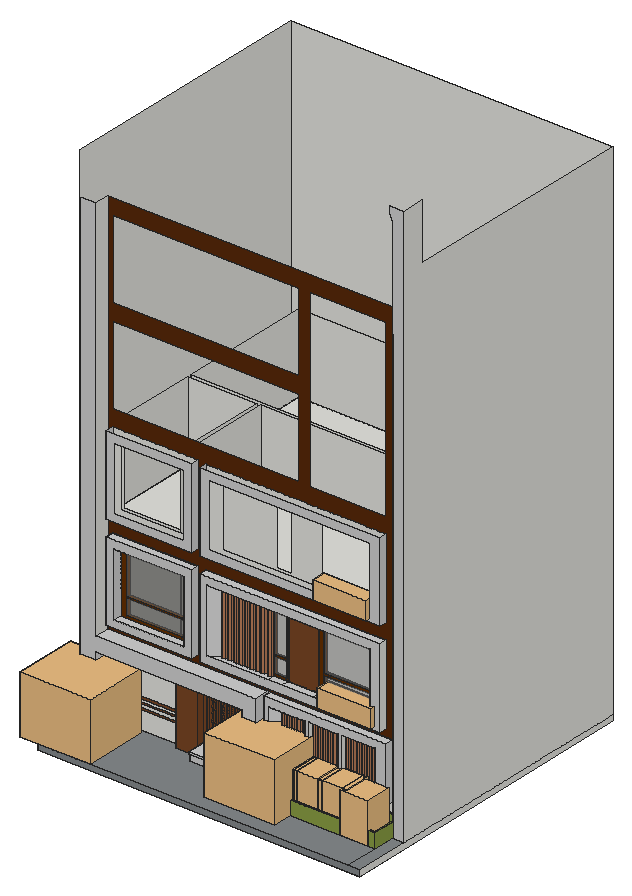
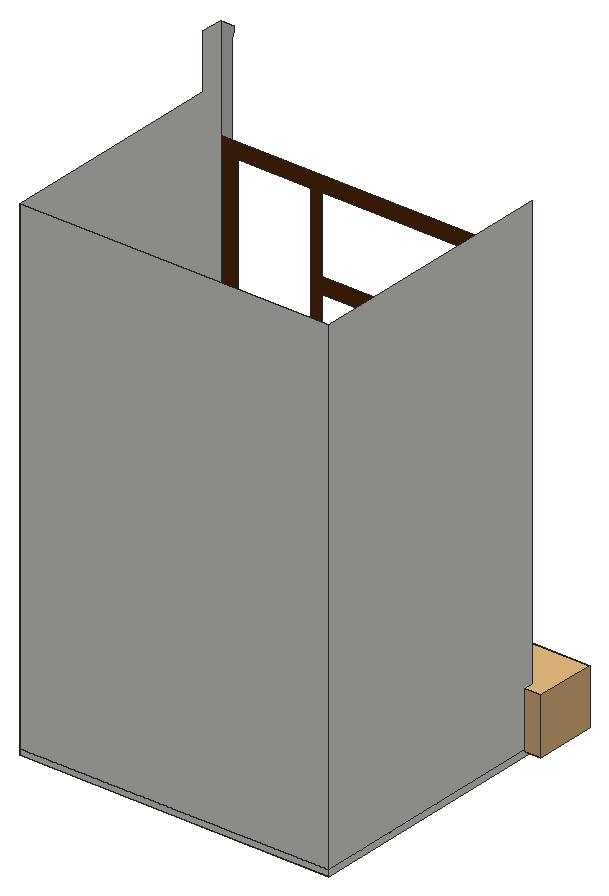
# SketchUp Ruby script. Lengths in inches.
U = 1.inch
M = Sketchup.active_model
def pt(a) = Geom::Point3d.new(a.map { |v| v * U })
def face(e, loops, mat)
  f = e.add_face(loops[0].map { |a| pt(a) })
  loops[1..].each { |l| e.add_face(l.map { |a| pt(a) }).erase! }
  f.material = f.back_material = mat if mat
  f
end
# faces: each face lists its corners as indices into pts; further lists are holes
def faces(e, pts, list, mat = nil) = list.each { |f| face(e, (f[0].is_a?(Array) ? f : [f]).map { |l| l.map { |i| pts[i] } }, mat) }
# xy, xz, yz: faces in a plane at the given z, y or x. An outline is a flat list of corners, or four numbers for a rectangle; further outlines are holes
def ring(l) = l.size == 4 ? [[l[0], l[1]], [l[2], l[1]], [l[2], l[3]], [l[0], l[3]]] : l.each_slice(2).to_a
def flat(e, list, mat, &to3) = list.each { |f| face(e, (f[0].is_a?(Array) ? f : [f]).map { |l| ring(l).map { |u, v| to3.(u, v) } }, mat) }
def xy(e, z, list, mat = nil) = flat(e, list, mat) { |x, y| [x, y, z] }
def xz(e, y, list, mat = nil) = flat(e, list, mat) { |x, z| [x, y, z] }
def yz(e, x, list, mat = nil) = flat(e, list, mat) { |y, z| [x, y, z] }
def lines(e, pts, list) = list.each { |a, b| e.add_line(pt(pts[a]), pt(pts[b])) }
# prism: a flat outline (further loops are holes) pulled along v
def prism(e, loops, v, mat = nil)
  f = face(e, loops, mat); d = Geom::Vector3d.new(v.map { |x| x * U })
  f.pushpull(f.normal.samedirection?(d) ? d.length : -d.length)
end
def box(e, o, s, mat = nil) = prism(e, [[o, [o[0] + s[0], o[1], o[2]], [o[0] + s[0], o[1] + s[1], o[2]], [o[0], o[1] + s[1], o[2]]]], [0, 0, s[2]], mat)
def at(x, y, z, deg = 0) = Geom::Transformation.translation(pt([x, y, z])) * Geom::Transformation.rotation(ORIGIN, Z_AXIS, deg.degrees)
def axes(o, x, y, z) = Geom::Transformation.new([*x, 0, *y, 0, *z, 0, *pt(o).to_a, 1])
def part(name) = M.definitions.add(name)
# library, detail: a bought-in or finely detailed component or shape, given as its bounding box
def library(name, o, s) = part(name).tap { |d| box(d.entities, o, s) }
def detail(e, o, s) = box(e.add_group.entities, o, s)
def put(e, d, t, mat = nil) = e.add_instance(d, t).tap { |i| i.material = mat if mat }
def group(e, t, mat = nil) = e.add_group.tap { |g| g.transformation = t; g.material = mat if mat }.entities
root = M.entities
M.materials.add("[Blacktop Old 01]").color = [132, 136, 139]
M.materials.add("[Blinds Vertical Stripe Gray]").color = [160, 160, 152]
M.materials.add("[Brick Antique 01]").color = [88, 41, 11]
M.materials.add("[Carrera Marble]").color = [207, 207, 207]
M.materials.add("[Color A08]").color = [102, 48, 0]
M.materials.add("[Grass Dark Green]").color = [106, 157, 55]
M.materials.add("[Grass Light Green]").color = [138, 158, 69]
M.materials.add("[Translucent Glass Gray]").color = [128, 128, 128]
M.materials["[Translucent Glass Gray]"].alpha = 0.5
M.materials.add("[Wood Veneer 01]").color = [120, 70, 37]
M.materials.add("[Wood Veneer 02]").color = [190, 128, 91]
c1 = library("Plante",[-44.1,-44.03,0.04],[106.77,95.72,88.04])
c2 = library("Flower",[-21.54,-20.15,0],[42.93,40.32,61.94])
c3 = library("Group\#7",[-1.66,-1.22,-7.38],[80.42,21.6,26.94])
c4 = part("Group\#4")
xy(c4.entities,0,[[0,0,42.75,0.0625],[0,0.0625,42.75,4.0625]],"[Color A08]")
xy(c4.entities,3.85,[[3.85,0,38.9,0.0625],[3.85,0.0625,38.9,4.0625]],"[Color A08]")
xy(c4.entities,34.99,[[3.85,0,38.9,0.0625],[3.85,0.0625,38.9,4.0625]],"[Color A08]")
xy(c4.entities,37.8125,[[3.85,0,38.9,0.0625],[3.85,0.0625,38.9,4.0625]],"[Color A08]")
xy(c4.entities,119.4,[[3.85,0,38.9,0.0625],[3.85,0.0625,38.9,4.0625]],"[Color A08]")
xy(c4.entities,123.25,[[0,0,42.75,0.0625],[0,0.0625,42.75,4.0625]],"[Color A08]")
xz(c4.entities,0,[[[0,0,42.75,123.25],[3.85,3.85,3.85,34.99,38.9,34.99,38.9,37.8125,3.85,37.8125,3.85,119.4,38.9,119.4,38.9,3.85]]],"[Color A08]")
xz(c4.entities,0.0625,[[[0,0,42.75,123.25],[3.85,3.85,3.85,34.99,38.9,34.99,38.9,37.8125,3.85,37.8125,3.85,119.4,38.9,119.4,38.9,3.85]]],"[Color A08]")
xz(c4.entities,0.0625,[[3.85,3.85,38.9,34.99],[3.85,37.8125,38.9,119.4]],"[Translucent Glass Gray]")
xz(c4.entities,4.0625,[[[0,0,42.75,123.25],[3.85,3.85,38.9,3.85,38.9,119.4,3.85,119.4,3.85,37.8125,38.9,37.8125,38.9,34.99,3.85,34.99]]],"[Color A08]")
yz(c4.entities,0,[[0,0,0.0625,123.25],[0.0625,0,4.0625,123.25]],"[Color A08]")
yz(c4.entities,3.85,[[0,3.85,0.0625,34.99],[0.0625,3.85,4.0625,34.99],[0,37.8125,0.0625,119.4],[0.0625,37.8125,4.0625,119.4]],"[Color A08]")
yz(c4.entities,38.9,[[0,3.85,0.0625,34.99],[0.0625,3.85,4.0625,34.99],[0,34.99,0.0625,37.8125],[0.0625,34.99,4.0625,37.8125],[0,37.8125,0.0625,119.4],
  [0.0625,37.8125,4.0625,119.4]],"[Color A08]")
yz(c4.entities,42.75,[[0,0,0.0625,123.25],[0.0625,0,4.0625,123.25]],"[Color A08]")
c5 = part("Group\#3")
xy(c5.entities,0,[[0,0,42.75,0.0625],[0,0.0625,42.75,4.0625]],"[Color A08]")
xy(c5.entities,3.85,[[3.85,0,38.9,0.0625],[3.85,0.0625,38.9,4.0625]],"[Color A08]")
xy(c5.entities,34.99,[[3.85,0,38.9,0.0625],[3.85,0.0625,38.9,4.0625]],"[Color A08]")
xy(c5.entities,37.8125,[[3.85,0,38.9,0.0625],[3.85,0.0625,38.9,4.0625]],"[Color A08]")
xy(c5.entities,119.4,[[3.85,0,38.9,0.0625],[3.85,0.0625,38.9,4.0625]],"[Color A08]")
xy(c5.entities,123.25,[[0,0,42.75,0.0625],[0,0.0625,42.75,4.0625]],"[Color A08]")
xz(c5.entities,0,[[[0,0,42.75,123.25],[3.85,3.85,3.85,34.99,38.9,34.99,38.9,37.8125,3.85,37.8125,3.85,119.4,38.9,119.4,38.9,3.85]]],"[Color A08]")
xz(c5.entities,0.0625,[[[0,0,42.75,123.25],[3.85,3.85,3.85,34.99,38.9,34.99,38.9,37.8125,3.85,37.8125,3.85,119.4,38.9,119.4,38.9,3.85]]],"[Color A08]")
xz(c5.entities,0.0625,[[3.85,3.85,38.9,34.99],[3.85,37.8125,38.9,119.4]],"[Translucent Glass Gray]")
xz(c5.entities,4.0625,[[[0,0,42.75,123.25],[3.85,3.85,38.9,3.85,38.9,119.4,3.85,119.4,3.85,37.8125,38.9,37.8125,38.9,34.99,3.85,34.99]]],"[Color A08]")
yz(c5.entities,0,[[0,0,0.0625,123.25],[0.0625,0,4.0625,123.25]],"[Color A08]")
yz(c5.entities,3.85,[[0,3.85,0.0625,34.99],[0.0625,3.85,4.0625,34.99],[0,37.8125,0.0625,119.4],[0.0625,37.8125,4.0625,119.4]],"[Color A08]")
yz(c5.entities,38.9,[[0,3.85,0.0625,34.99],[0.0625,3.85,4.0625,34.99],[0,34.99,0.0625,37.8125],[0.0625,34.99,4.0625,37.8125],[0,37.8125,0.0625,119.4],
  [0.0625,37.8125,4.0625,119.4]],"[Color A08]")
yz(c5.entities,42.75,[[0,0,0.0625,123.25],[0.0625,0,4.0625,123.25]],"[Color A08]")
xy(root,0,[[0,0,487.5,480]])
xy(root,9,[[[0,79.3125,0,480,487.5,480,487.5,83.875,470.5,83.875,470.5,252.8125,135.23,252.8125,135.23,108.75,470.5,108.75,470.5,102.75,24.5,102.75,24.5,108.75,129.23,108.75,129.23,252.8125,24.5,252.8125,24.5,79.3125],[24.5,258.8125,337.8125,463],[343.8125,258.8125,470.5,463]],[167.61,79.3125,267.125,102.75],[24.5,108.75,129.23,252.8125],[135.23,108.75,470.5,252.8125],[24.5,258.8125,337.8125,463],
  [343.8125,258.8125,470.5,463]])
xy(root,9,[[0,0,0,79.3125,24.5,79.3125,24.5,102.75,133.26,102.75,133.26,94.375,167.61,94.375,167.61,79.3125,267.125,79.3125,267.125,51.24,470.5,51.24,470.5,0],[470.5,0,487.5,83.875]],"[Blacktop Old 01]")
xy(root,9,[[269.4375,53.55,468.1875,100.4375]],"[Grass Dark Green]")
xy(root,9,[[[267.125,51.24,470.5,102.75],[269.4375,53.55,468.1875,100.4375]]],"[Grass Light Green]")
xy(root,9,[[133.26,94.375,167.61,102.75]],"[Wood Veneer 01]")
xy(root,20.625,[[167.18,76.625,245.72,79.3125],[167.18,79.3125,167.61,94.375],[167.61,79.3125,245.72,102.75]])
xy(root,20.625,[[167.18,94.375,167.61,102.75]],"[Wood Veneer 01]")
xy(root,23.1875,[[167.18,76.625,245.72,102.75]],"[Carrera Marble]")
xy(root,30.25,[[[267.125,51.24,470.5,102.75],[269.4375,53.55,468.1875,100.4375]]],"[Grass Light Green]")
xy(root,45.0625,[[270,90.75,455.5,102.75]],"[Carrera Marble]")
xy(root,62.0625,[[[277.72,90.75,332.83,90.75,332.83,102.75,290.32,102.75],[293.9375,94.8,298.625,100.49],[301.75,94.8,306.4375,100.49],[309.5625,94.8,314.25,100.49],[317.375,94.8,322.0625,100.49],[325.1875,94.8,329.875,100.49]],[[338.64,90.75,381.71,102.75],[340.8125,94.8,345.5,100.49],[348.625,94.8,353.3125,100.49],[356.4375,94.8,361.125,100.49],[364.25,94.8,368.9375,100.49],[372.0625,94.8,376.75,100.49]],[[387.52,90.75,438.5,102.75],[390.625,94.8,395.3125,100.49],[399,94.8,403.6875,100.49],[407.1875,94.8,411.875,100.49],[415.4375,94.8,420.125,100.49],[422.875,94.8,427.5625,100.49],[430.875,94.8,435.5625,100.49]],[333,94.8,337.6875,100.49],[381.71,94.8,384.5625,100.49],
  [438.5,94.8,439.25,100.49],[442.375,94.8,447.0625,100.49],[450.1875,94.8,454.875,100.49]])
xy(root,62.0625,[[293.9375,94.8,298.625,100.49],[301.75,94.8,306.4375,100.49],[309.5625,94.8,314.25,100.49],[317.375,94.8,322.0625,100.49],[325.1875,94.8,329.875,100.49],
  [340.8125,94.8,345.5,100.49],[348.625,94.8,353.3125,100.49],[356.4375,94.8,361.125,100.49],[364.25,94.8,368.9375,100.49],[372.0625,94.8,376.75,100.49],
  [390.625,94.8,395.3125,100.49],[399,94.8,403.6875,100.49],[407.1875,94.8,411.875,100.49],[415.4375,94.8,420.125,100.49],[422.875,94.8,427.5625,100.49],
  [430.875,94.8,435.5625,100.49]],"[Wood Veneer 02]")
xy(root,97.5625,[[343.8125,258.8125,470.5,463]])
xy(root,107,[[24.5,79.3125,24.5,102.75,133.26,102.75,133.26,94.375,167.18,94.375,167.18,102.75,245.72,102.75,245.72,79.3125]],"[Carrera Marble]")
xy(root,107,[[133.26,94.375,167.18,102.75]],"[Wood Veneer 01]")
xy(root,117,[[[277.72,90.75,290.32,102.75,332.83,102.75,332.83,90.75],[301.75,94.8,306.4375,100.49],[325.1875,94.8,329.875,100.49]],[[338.64,90.75,381.71,102.75],[340.8125,94.8,345.5,100.49]],[[387.52,90.75,438.5,102.75],[399,94.8,403.6875,100.49],[415.4375,94.8,420.125,100.49]]],"[Carrera Marble]")
xy(root,117.0625,[[293.9375,94.8,298.625,100.49]],"[Wood Veneer 02]")
xy(root,117.3125,[[356.4375,94.8,361.125,100.49]],"[Wood Veneer 02]")
xy(root,117.4375,[[390.625,94.8,395.3125,100.49]],"[Wood Veneer 02]")
xy(root,117.75,[[309.5625,94.8,314.25,100.49]],"[Wood Veneer 02]")
xy(root,118,[[372.0625,94.8,376.75,100.49]],"[Wood Veneer 02]")
xy(root,118.1875,[[407.1875,94.8,411.875,100.49]],"[Wood Veneer 02]")
xy(root,118.3125,[[317.375,94.8,322.0625,100.49]],"[Wood Veneer 02]")
xy(root,119.375,[[348.625,94.8,353.3125,100.49]],"[Wood Veneer 02]")
xy(root,120.75,[[364.25,94.8,368.9375,100.49]],"[Wood Veneer 02]")
xy(root,121,[[422.875,94.8,427.5625,100.49]],"[Wood Veneer 02]")
xy(root,121.5,[[430.875,94.8,435.5625,100.49]],"[Wood Veneer 02]")
xy(root,123,[[24.5,258.8125,337.8125,463]])
xy(root,129,[[24.5,258.8125,337.8125,463]])
xy(root,129,[[24.5,79.3125,267.125,102.75],[270,90.75,455.5,102.75]],"[Carrera Marble]")
xy(root,136.8125,[[135.23,108.75,470.5,252.8125]])
xy(root,141,[[24.5,108.75,129.23,252.8125],[135.23,108.75,470.5,252.8125],[343.8125,258.8125,470.5,463]])
xy(root,141,[[31.1875,90.75,160.25,102.75],[173,90.75,445.6875,102.75]],"[Carrera Marble]")
xy(root,153,[[43.1875,102.75,148.25,108.75],[276.03,102.75,297.76,108.75],[344.2,102.75,431.1875,108.75]])
xy(root,153,[[43.1875,90.75,148.25,102.75],[184.1,90.75,276.03,90.75,276.03,98.6875,270.24,98.6875,270.24,102.75,265.41,102.75,265.41,98.6875,259.61,98.6875,259.61,102.75,256.97,102.75,256.97,98.6875,251.18,98.6875,251.18,102.75,248.53,102.75,248.53,98.6875,242.74,98.6875,242.74,102.75,240.09,102.75,240.09,98.6875,234.3,98.6875,234.3,102.75,231.66,102.75,231.66,98.6875,225.86,98.6875,225.86,102.75,223.22,102.75,223.22,98.6875,217.43,98.6875,217.43,102.75,214.78,102.75,214.78,98.6875,208.99,98.6875,208.99,102.75,206.34,102.75,206.34,98.6875,200.55,98.6875,200.55,102.75,198.8125,102.75],[276.03,90.75,297.76,102.75],[297.76,90.75,344.2,102.75],[344.2,90.75,431.1875,102.75]],"[Carrera Marble]")
xy(root,153,[[200.55,98.6875,206.34,102.75],[208.99,98.6875,214.78,102.75],[217.43,98.6875,223.22,102.75],[225.86,98.6875,231.66,102.75],[234.3,98.6875,240.09,102.75],
  [242.74,98.6875,248.53,102.75],[251.18,98.6875,256.97,102.75],[259.61,98.6875,265.41,102.75],[270.24,98.6875,276.03,102.75]],"[Wood Veneer 02]")
xy(root,249,[[43.1875,90.75,148.25,102.75],[43.1875,102.75,148.25,108.75],[276.03,102.75,297.76,108.75],[344.2,102.75,431.1875,108.75]])
xy(root,249,[[184.1,90.75,198.8125,102.75,200.55,102.75,200.55,98.6875,206.34,98.6875,206.34,102.75,208.99,102.75,208.99,98.6875,214.78,98.6875,214.78,102.75,217.43,102.75,217.43,98.6875,223.22,98.6875,223.22,102.75,225.86,102.75,225.86,98.6875,231.66,98.6875,231.66,102.75,234.3,102.75,234.3,98.6875,240.09,98.6875,240.09,102.75,242.74,102.75,242.74,98.6875,248.53,98.6875,248.53,102.75,251.18,102.75,251.18,98.6875,256.97,98.6875,256.97,102.75,259.61,102.75,259.61,98.6875,265.41,98.6875,265.41,102.75,270.24,102.75,270.24,98.6875,276.03,98.6875,276.03,90.75],[276.03,90.75,297.76,102.75],[297.76,90.75,344.2,102.75],[344.2,90.75,431.1875,102.75]],"[Carrera Marble]")
xy(root,249,[[200.55,98.6875,206.34,102.75],[208.99,98.6875,214.78,102.75],[217.43,98.6875,223.22,102.75],[225.86,98.6875,231.66,102.75],[234.3,98.6875,240.09,102.75],
  [242.74,98.6875,248.53,102.75],[251.18,98.6875,256.97,102.75],[259.61,98.6875,265.41,102.75],[270.24,98.6875,276.03,102.75]],"[Wood Veneer 02]")
xy(root,261,[[31.1875,90.75,160.25,102.75],[173,90.75,445.6875,102.75]],"[Carrera Marble]")
xy(root,279,[[24.5,258.8125,337.8125,463]])
xy(root,280.5625,[[343.8125,258.8125,470.5,463]])
xy(root,285,[[173,90.75,445.6875,102.75],[24.5,108.75,129.23,252.8125],[135.23,108.75,470.5,252.8125],[24.5,258.8125,337.8125,463],[343.8125,258.8125,470.5,463]])
xy(root,285,[[31.1875,90.75,160.25,102.75]],"[Carrera Marble]")
xz(root,0,[[0,0,487.5,9]],"[Blacktop Old 01]")
xz(root,51.24,[[267.125,9,470.5,30.25]],"[Grass Light Green]")
xz(root,53.55,[[269.4375,9,468.1875,30.25]],"[Grass Light Green]")
xz(root,76.625,[[167.18,20.625,245.72,23.1875]],"[Carrera Marble]")
xz(root,79.3125,[[0,9,24.5,9,24.5,107,245.72,107,245.72,20.625,167.61,20.625,167.61,9,267.125,9,267.125,129,24.5,129,24.5,717,0,717]],"[Carrera Marble]")
xz(root,83.875,[[470.5,9,487.5,9,487.5,865.9375,466.875,865.9375,466.875,856.375,470.5,845.4375]],"[Carrera Marble]")
xz(root,90.75,[[[270,45.0625,455.5,129],[277.72,62.0625,332.83,117],[387.52,62.0625,438.5,117],[338.64,62.0625,381.71,117]],[[31.1875,141,160.25,261],[43.1875,153,148.25,249]],[[173,141,445.6875,261],[184.1,153,431.1875,249]],[[31.1875,285,160.25,405],[43.1875,297,148.25,393]],[[173,285,445.6875,405],[185.91,297,431.1875,393]]],"[Carrera Marble]")
xz(root,94.375,[[133.26,9,167.61,9,167.61,20.625,167.18,20.625,167.18,107,133.26,107]],"[Wood Veneer 01]")
xz(root,94.8,[[293.9375,62.0625,298.625,117.0625],[301.75,62.0625,306.4375,117],[309.5625,62.0625,314.25,117.75],[317.375,62.0625,322.0625,118.3125],[325.1875,62.0625,329.875,117],
  [340.8125,62.0625,345.5,117],[348.625,62.0625,353.3125,119.375],[356.4375,62.0625,361.125,117.3125],[364.25,62.0625,368.9375,120.75],[372.0625,62.0625,376.75,118],
  [390.625,62.0625,395.3125,117.4375],[399,62.0625,403.6875,117],[407.1875,62.0625,411.875,118.1875],[415.4375,62.0625,420.125,117],[422.875,62.0625,427.5625,121],
  [430.875,62.0625,435.5625,121.5]],"[Wood Veneer 02]")
xz(root,98.6875,[[200.55,153,206.34,249],[208.99,153,214.78,249],[217.43,153,223.22,249],[225.86,153,231.66,249],[234.3,153,240.09,249],
  [242.74,153,248.53,249],[251.18,153,256.97,249],[259.61,153,265.41,249],[270.24,153,276.03,249]],"[Wood Veneer 02]")
xz(root,100.4375,[[269.4375,9,468.1875,30.25]],"[Grass Light Green]")
xz(root,100.49,[[293.9375,62.0625,298.625,117.0625],[301.75,62.0625,306.4375,117],[309.5625,62.0625,314.25,117.75],[317.375,62.0625,322.0625,118.3125],[325.1875,62.0625,329.875,117],
  [340.8125,62.0625,345.5,117],[348.625,62.0625,353.3125,119.375],[356.4375,62.0625,361.125,117.3125],[364.25,62.0625,368.9375,120.75],[372.0625,62.0625,376.75,118],
  [390.625,62.0625,395.3125,117.4375],[399,62.0625,403.6875,117],[407.1875,62.0625,411.875,118.1875],[415.4375,62.0625,420.125,117],[422.875,62.0625,427.5625,121],
  [430.875,62.0625,435.5625,121.5]],"[Wood Veneer 02]")
xz(root,102.75,[[167.61,9,167.61,20.625,245.72,20.625,245.72,107,24.5,107,24.5,129,267.125,129,267.125,9],[24.5,9,133.26,35.71],[167.18,20.625,245.72,23.1875],[267.125,30.25,470.5,30.25,470.5,129,455.5,129,455.5,45.0625,270,45.0625,270,129,267.125,129],[24.5,39.45,133.26,43.82],
  [[270,45.0625,455.5,129],[290.32,62.0625,332.83,62.0625,332.83,117,338.64,117,338.64,62.0625,381.71,62.0625,381.71,117,290.32,117],[387.52,62.0625,438.5,117]],[24.5,47.5625,133.26,51.38],[24.5,55.125,133.26,92.51],[24.5,96.25,133.26,107],[[31.1875,141,160.25,261],[43.1875,153,148.25,249]],
  [[173,141,445.6875,261],[198.8125,153,431.1875,249]],[[31.1875,285,160.25,405],[43.1875,297,148.25,393]],[[173,285,445.6875,405],[198.8125,297,431.1875,393]]])
xz(root,102.75,[[[24.5,129,470.5,717],[31.25,573,312.9375,693],[31.25,429,312.9375,549],[173,285,445.6875,405],[173,141,445.6875,261],[330,429,445.6875,693],[31.1875,285,160.25,405],[31.1875,141,160.25,261]]],"[Brick Antique 01]")
xz(root,102.75,[[267.125,9,470.5,30.25]],"[Grass Light Green]")
xz(root,102.75,[[133.26,9,133.26,107,167.18,107,167.18,20.625,167.61,20.625,167.61,9],[167.18,23.1875,171.83,107],[171.83,23.1875,174.2,107],[174.2,23.1875,176.58,107],[176.58,23.1875,178.95,107],
  [178.95,23.1875,181.33,107],[181.33,23.1875,183.7,107],[183.7,23.1875,186.08,107],[186.08,23.1875,188.45,107],[188.45,23.1875,190.83,107],
  [190.83,23.1875,193.2,107],[193.2,23.1875,195.58,107],[195.58,23.1875,197.95,107],[197.95,23.1875,200.33,107],[200.33,23.1875,202.7,107],
  [202.7,23.1875,205.08,107],[205.08,23.1875,207.45,107],[207.45,23.1875,209.83,107],[209.83,23.1875,212.2,107],[212.2,23.1875,214.58,107],
  [214.58,23.1875,216.95,107],[216.95,23.1875,219.33,107],[219.33,23.1875,221.7,107],[221.7,23.1875,224.08,107],[224.08,23.1875,226.45,107],
  [226.45,23.1875,228.83,107],[228.83,23.1875,231.2,107],[231.2,23.1875,233.58,107],[233.58,23.1875,235.7,107],[235.7,23.1875,237.83,107],
  [237.83,23.1875,239.64,107],[239.64,23.1875,241.95,107],[241.95,23.1875,243.84,107],[243.84,23.1875,245.72,107],[24.5,35.71,133.26,39.45],
  [24.5,43.82,133.26,47.5625],[24.5,51.38,133.26,55.125],[290.32,62.0625,332.83,117],[338.64,62.0625,381.71,117],[387.52,62.0625,438.5,117],
  [24.5,92.51,133.26,96.25],[198.8125,153,200.55,249],[206.34,153,208.99,249],[214.78,153,217.43,249],[223.22,153,225.86,249],
  [231.66,153,234.3,249],[240.09,153,242.74,249],[248.53,153,251.18,249],[256.97,153,259.61,249],[265.41,153,270.24,249],
  [297.76,153,344.2,249]],"[Wood Veneer 01]")
xz(root,102.75,[[200.55,153,206.34,249],[208.99,153,214.78,249],[217.43,153,223.22,249],[225.86,153,231.66,249],[234.3,153,240.09,249],
  [242.74,153,248.53,249],[251.18,153,256.97,249],[259.61,153,265.41,249],[270.24,153,276.03,249]],"[Wood Veneer 02]")
xz(root,108.75,[[24.5,9,129.23,129],[135.23,9,470.5,129],[24.5,129,129.23,141],[135.23,129,470.5,136.8125],[135.23,136.8125,470.5,141],
  [24.5,141,24.5,261,129.23,261,129.23,249,43.1875,249,43.1875,153,129.23,153,129.23,141],[[135.23,141,135.23,153,148.25,153,148.25,249,135.23,249,135.23,261,470.5,261,470.5,141],[344.2,153,431.1875,249],[276.03,153,297.76,249]],[24.5,261,129.23,285],[135.23,261,470.5,285],[24.5,285,24.5,405,129.23,405,129.23,393,43.1875,393,43.1875,297,129.23,297,129.23,285],
  [[135.23,285,135.23,297,148.25,297,148.25,393,135.23,393,135.23,405,470.5,405,470.5,285],[344.2,297,431.1875,393],[276.03,297,297.76,393]]])
xz(root,108.75,[[43.1875,153,129.23,249],[129.23,153,135.23,249],[135.23,153,148.25,249]],"[Blinds Vertical Stripe Gray]")
xz(root,252.8125,[[24.5,9,129.23,129],[135.23,9,470.5,129],[24.5,129,129.23,141],[135.23,129,470.5,136.8125],[135.23,136.8125,470.5,141],
  [24.5,141,129.23,261],[135.23,141,470.5,261],[24.5,261,129.23,285],[135.23,261,470.5,285],[24.5,285,129.23,405],
  [135.23,285,470.5,405]])
xz(root,258.8125,[[24.5,9,337.8125,123],[343.8125,9,470.5,97.5625],[343.8125,97.5625,461.125,129],[461.125,97.5625,470.5,129],[24.5,123,337.8125,129],
  [24.5,129,337.8125,141],[343.8125,129,461.125,141],[461.125,129,470.5,141],[24.5,141,337.8125,261],[343.8125,141,470.5,261],
  [24.5,261,337.8125,279],[343.8125,261,470.5,280.5625],[24.5,279,337.8125,285],[343.8125,280.5625,455.76,285],[455.76,280.5625,463.01,285],
  [463.01,280.5625,470.5,285],[24.5,285,337.8125,405],[343.8125,285,470.5,405]])
xz(root,463,[[24.5,9,337.8125,123],[343.8125,9,470.5,97.5625],[343.8125,97.5625,470.5,129],[24.5,123,37.125,129],[37.125,123,337.8125,129],
  [24.5,129,337.8125,141],[343.8125,129,470.5,141],[24.5,141,337.8125,261],[343.8125,141,470.5,261],[24.5,261,337.8125,279],
  [343.8125,261,470.5,280.5625],[24.5,279,45.88,285],[45.88,279,56.88,285],[56.88,279,337.8125,285],[343.8125,280.5625,470.5,285],
  [24.5,285,337.8125,405],[343.8125,285,470.5,405]])
xz(root,480,[[0,0,487.5,9],[0,9,487.5,780.4375]])
yz(root,0,[[0,0,480,9],[79.3125,9,480,780.4375]])
yz(root,24.5,[[102.75,9,108.75,129],[108.75,9,252.8125,129],[258.8125,9,463,123],[258.8125,123,463,129],[79.3125,129,102.75,717],
  [102.75,129,108.75,141],[108.75,129,252.8125,141],[258.8125,129,463,141],[102.75,141,108.75,261],[108.75,141,252.8125,261],
  [258.8125,141,463,261],[102.75,261,108.75,285],[108.75,261,252.8125,285],[258.8125,261,463,279],[258.8125,279,463,285],
  [102.75,285,108.75,405],[108.75,285,252.8125,405],[258.8125,285,463,405]])
yz(root,24.5,[[79.3125,9,102.75,107]],"[Carrera Marble]")
yz(root,31.1875,[[90.75,141,102.75,261],[90.75,285,102.75,405]],"[Carrera Marble]")
yz(root,43.1875,[[102.75,153,108.75,249]])
yz(root,43.1875,[[90.75,153,102.75,249]],"[Carrera Marble]")
yz(root,129.23,[[108.75,9,252.8125,129],[108.75,129,252.8125,141],[108.75,141,252.8125,261],[108.75,261,252.8125,285],[108.75,285,252.8125,405]])
yz(root,133.26,[[94.375,9,102.75,35.71],[94.375,35.71,102.75,39.45],[94.375,39.45,102.75,43.82],[94.375,43.82,102.75,47.5625],[94.375,47.5625,102.75,51.38],
  [94.375,51.38,102.75,55.125],[94.375,55.125,102.75,92.51],[94.375,92.51,102.75,96.25],[94.375,96.25,102.75,107]],"[Wood Veneer 01]")
yz(root,135.23,[[108.75,9,252.8125,129],[108.75,129,252.8125,136.8125],[108.75,136.8125,117.32,141],[117.32,136.8125,123.25,141],[123.25,136.8125,252.8125,141],
  [108.75,141,252.8125,261],[108.75,261,252.8125,285],[108.75,285,252.8125,405]])
yz(root,148.25,[[102.75,153,108.75,249]])
yz(root,148.25,[[90.75,153,102.75,249]],"[Carrera Marble]")
yz(root,160.25,[[90.75,141,102.75,261],[90.75,285,102.75,405]],"[Carrera Marble]")
yz(root,167.18,[[76.625,20.625,94.375,23.1875]],"[Carrera Marble]")
yz(root,167.18,[[94.375,20.625,102.75,23.1875],[94.375,23.1875,102.75,107]],"[Wood Veneer 01]")
yz(root,167.61,[[79.3125,9,94.375,20.625]],"[Carrera Marble]")
yz(root,167.61,[[94.375,9,102.75,20.625]],"[Wood Veneer 01]")
yz(root,173,[[90.75,141,102.75,261],[90.75,285,102.75,405]],"[Carrera Marble]")
yz(root,200.55,[[98.6875,153,102.75,249]],"[Wood Veneer 02]")
yz(root,206.34,[[98.6875,153,102.75,249]],"[Wood Veneer 02]")
yz(root,208.99,[[98.6875,153,102.75,249]],"[Wood Veneer 02]")
yz(root,214.78,[[98.6875,153,102.75,249]],"[Wood Veneer 02]")
yz(root,217.43,[[98.6875,153,102.75,249]],"[Wood Veneer 02]")
yz(root,223.22,[[98.6875,153,102.75,249]],"[Wood Veneer 02]")
yz(root,225.86,[[98.6875,153,102.75,249]],"[Wood Veneer 02]")
yz(root,231.66,[[98.6875,153,102.75,249]],"[Wood Veneer 02]")
yz(root,234.3,[[98.6875,153,102.75,249]],"[Wood Veneer 02]")
yz(root,240.09,[[98.6875,153,102.75,249]],"[Wood Veneer 02]")
yz(root,242.74,[[98.6875,153,102.75,249]],"[Wood Veneer 02]")
yz(root,245.72,[[76.625,20.625,79.3125,23.1875],[79.3125,20.625,102.75,23.1875]])
yz(root,245.72,[[79.3125,23.1875,102.75,107]],"[Carrera Marble]")
yz(root,248.53,[[98.6875,153,102.75,249]],"[Wood Veneer 02]")
yz(root,251.18,[[98.6875,153,102.75,249]],"[Wood Veneer 02]")
yz(root,256.97,[[98.6875,153,102.75,249]],"[Wood Veneer 02]")
yz(root,259.61,[[98.6875,153,102.75,249]],"[Wood Veneer 02]")
yz(root,265.41,[[98.6875,153,102.75,249]],"[Wood Veneer 02]")
yz(root,267.125,[[79.3125,30.25,102.75,129]],"[Carrera Marble]")
yz(root,267.125,[[51.24,9,79.3125,30.25],[79.3125,9,102.75,30.25]],"[Grass Light Green]")
yz(root,269.4375,[[53.55,9,79.3125,30.25],[79.3125,9,100.4375,30.25]],"[Grass Light Green]")
yz(root,270,[[90.75,45.0625,102.75,129]],"[Carrera Marble]")
yz(root,270.24,[[98.6875,153,102.75,249]],"[Wood Veneer 02]")
yz(root,276.03,[[102.75,153,108.75,249]],"[Wood Veneer 01]")
yz(root,276.03,[[98.6875,153,102.75,249]],"[Wood Veneer 02]")
yz(root,293.9375,[[94.8,62.0625,100.49,117.0625]],"[Wood Veneer 02]")
yz(root,297.76,[[102.75,153,108.75,249]],"[Wood Veneer 01]")
yz(root,298.625,[[94.8,62.0625,100.49,117.0625]],"[Wood Veneer 02]")
yz(root,301.75,[[94.8,62.0625,100.49,117]],"[Wood Veneer 02]")
yz(root,306.4375,[[94.8,62.0625,100.49,117]],"[Wood Veneer 02]")
yz(root,309.5625,[[94.8,62.0625,100.49,117.75]],"[Wood Veneer 02]")
yz(root,314.25,[[94.8,62.0625,100.49,117.75]],"[Wood Veneer 02]")
yz(root,317.375,[[94.8,62.0625,100.49,118.3125]],"[Wood Veneer 02]")
yz(root,322.0625,[[94.8,62.0625,100.49,118.3125]],"[Wood Veneer 02]")
yz(root,325.1875,[[94.8,62.0625,100.49,117]],"[Wood Veneer 02]")
yz(root,329.875,[[94.8,62.0625,100.49,117]],"[Wood Veneer 02]")
yz(root,332.83,[[90.75,62.0625,102.75,117]])
yz(root,337.8125,[[258.8125,9,463,123],[258.8125,123,463,129],[258.8125,129,463,141],[258.8125,141,463,261],[258.8125,261,463,279],
  [258.8125,279,463,285],[258.8125,285,463,405]])
yz(root,338.64,[[90.75,62.0625,102.75,117]])
yz(root,340.8125,[[94.8,62.0625,100.49,117]],"[Wood Veneer 02]")
yz(root,343.8125,[[258.8125,9,463,97.5625],[258.8125,97.5625,463,129],[258.8125,129,463,141],[258.8125,141,463,261],[258.8125,261,463,280.5625],
  [258.8125,280.5625,463,285],[258.8125,285,463,405]])
yz(root,344.2,[[102.75,153,108.75,249]],"[Wood Veneer 01]")
yz(root,345.5,[[94.8,62.0625,100.49,117]],"[Wood Veneer 02]")
yz(root,348.625,[[94.8,62.0625,100.49,119.375]],"[Wood Veneer 02]")
yz(root,353.3125,[[94.8,62.0625,100.49,119.375]],"[Wood Veneer 02]")
yz(root,356.4375,[[94.8,62.0625,100.49,117.3125]],"[Wood Veneer 02]")
yz(root,361.125,[[94.8,62.0625,100.49,117.3125]],"[Wood Veneer 02]")
yz(root,364.25,[[94.8,62.0625,100.49,120.75]],"[Wood Veneer 02]")
yz(root,368.9375,[[94.8,62.0625,100.49,120.75]],"[Wood Veneer 02]")
yz(root,372.0625,[[94.8,62.0625,100.49,118]],"[Wood Veneer 02]")
yz(root,376.75,[[94.8,62.0625,100.49,118]],"[Wood Veneer 02]")
yz(root,381.71,[[90.75,62.0625,102.75,117]])
yz(root,387.52,[[90.75,62.0625,102.75,117]])
yz(root,390.625,[[94.8,62.0625,100.49,117.4375]],"[Wood Veneer 02]")
yz(root,395.3125,[[94.8,62.0625,100.49,117.4375]],"[Wood Veneer 02]")
yz(root,399,[[94.8,62.0625,100.49,117]],"[Wood Veneer 02]")
yz(root,403.6875,[[94.8,62.0625,100.49,117]],"[Wood Veneer 02]")
yz(root,407.1875,[[94.8,62.0625,100.49,118.1875]],"[Wood Veneer 02]")
yz(root,411.875,[[94.8,62.0625,100.49,118.1875]],"[Wood Veneer 02]")
yz(root,415.4375,[[94.8,62.0625,100.49,117]],"[Wood Veneer 02]")
yz(root,420.125,[[94.8,62.0625,100.49,117]],"[Wood Veneer 02]")
yz(root,422.875,[[94.8,62.0625,100.49,121]],"[Wood Veneer 02]")
yz(root,427.5625,[[94.8,62.0625,100.49,121]],"[Wood Veneer 02]")
yz(root,430.875,[[94.8,62.0625,100.49,121.5]],"[Wood Veneer 02]")
yz(root,431.1875,[[102.75,153,108.75,249]])
yz(root,431.1875,[[90.75,153,102.75,249]],"[Carrera Marble]")
yz(root,435.5625,[[94.8,62.0625,100.49,121.5]],"[Wood Veneer 02]")
yz(root,438.5,[[90.75,62.0625,102.75,117]])
yz(root,445.6875,[[90.75,141,102.75,261]])
yz(root,445.6875,[[90.75,285,102.75,405]],"[Carrera Marble]")
yz(root,455.5,[[90.75,45.0625,102.75,129]],"[Carrera Marble]")
yz(root,468.1875,[[53.55,9,83.875,30.25],[83.875,9,100.4375,30.25]],"[Grass Light Green]")
yz(root,470.5,[[102.75,9,108.75,129],[108.75,9,252.8125,129],[258.8125,9,463,97.5625],[83.875,30.25,102.75,693],[258.8125,97.5625,463,129],
  [102.75,129,108.75,141],[108.75,129,252.8125,136.8125],[258.8125,129,463,141],[108.75,136.8125,252.8125,141],[102.75,141,108.75,261],
  [108.75,141,252.8125,261],[258.8125,141,463,261],[102.75,261,108.75,285],[108.75,261,252.8125,285],[258.8125,261,463,280.5625],
  [258.8125,280.5625,463,285],[102.75,285,108.75,405],[108.75,285,252.8125,405],[258.8125,285,463,405]])
yz(root,470.5,[[51.24,9,83.875,30.25],[83.875,9,102.75,30.25]],"[Grass Light Green]")
yz(root,487.5,[[0,0,480,9],[83.875,9,480,9,480,780.4375,118.83,780.4375,118.83,865.9375,83.875,865.9375]])
p = [[277.72,90.75,62.0625],[290.32,102.75,62.0625],[290.32,102.75,117],[277.72,90.75,117],[184.1,90.75,153],[198.8125,102.75,153],
  [198.8125,102.75,249],[184.1,90.75,249],[387.52,102.75,117],[381.71,102.75,117],[133.26,102.75,9],[133.26,102.75,2.0625]]
faces(root,p,[[0,1,2,3],[4,5,6,7]],"[Carrera Marble]")
lines(root,p,[[8,9],[10,11]])
put(root,c1,at(16.9,44.03,8.96))
put(root,c2,at(327.6,74.44,9))
put(root,c2,at(365.91,74.44,9))
put(root,c2,at(402.85,74.44,9))
put(root,c2,at(438.33,70.67,9))
put(root,c1,at(278.86,65.875,8.96))
put(root,c3,at(357.94,85.44,152.8))
put(root,c4,axes([275.71,102.75,153],[0.51591,0,0],[0,0.7,0],[0,0,0.777]))
put(root,c5,axes([43.1875,102.64,153],[2.4576,0,0],[0,1.687,0],[0,0,0.777]))
put(root,c5,axes([344.2,102.75,153],[2.03468,0,0],[0,1.14716,0],[0,0,0.7789]))
put(root,c3,at(350.23,86.42,296.92))
